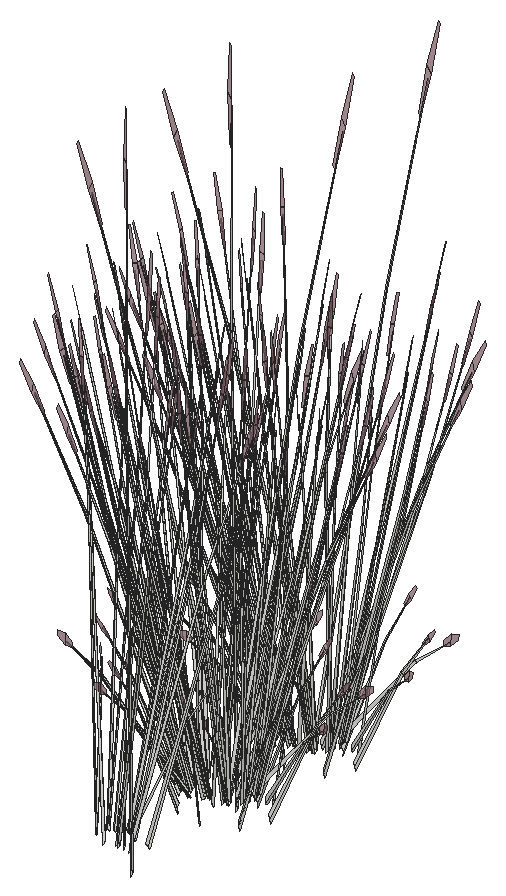
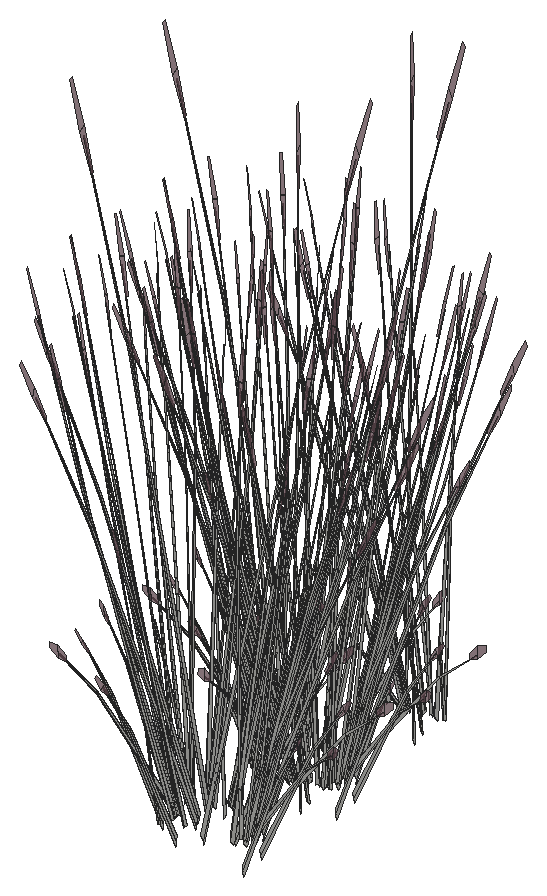
# SketchUp Ruby script. Lengths in inches.
U = 1.inch
M = Sketchup.active_model
def pt(a) = Geom::Point3d.new(a.map { |v| v * U })
def face(e, loops, mat)
  f = e.add_face(loops[0].map { |a| pt(a) })
  loops[1..].each { |l| e.add_face(l.map { |a| pt(a) }).erase! }
  f.material = f.back_material = mat if mat
  f
end
# faces: each face lists its corners as indices into pts; further lists are holes
def faces(e, pts, list, mat = nil) = list.each { |f| face(e, (f[0].is_a?(Array) ? f : [f]).map { |l| l.map { |i| pts[i] } }, mat) }
# xy, xz, yz: faces in a plane at the given z, y or x. An outline is a flat list of corners, or four numbers for a rectangle; further outlines are holes
def ring(l) = l.size == 4 ? [[l[0], l[1]], [l[2], l[1]], [l[2], l[3]], [l[0], l[3]]] : l.each_slice(2).to_a
def flat(e, list, mat, &to3) = list.each { |f| face(e, (f[0].is_a?(Array) ? f : [f]).map { |l| ring(l).map { |u, v| to3.(u, v) } }, mat) }
def xy(e, z, list, mat = nil) = flat(e, list, mat) { |x, y| [x, y, z] }
def xz(e, y, list, mat = nil) = flat(e, list, mat) { |x, z| [x, y, z] }
def yz(e, x, list, mat = nil) = flat(e, list, mat) { |y, z| [x, y, z] }
def lines(e, pts, list) = list.each { |a, b| e.add_line(pt(pts[a]), pt(pts[b])) }
# prism: a flat outline (further loops are holes) pulled along v
def prism(e, loops, v, mat = nil)
  f = face(e, loops, mat); d = Geom::Vector3d.new(v.map { |x| x * U })
  f.pushpull(f.normal.samedirection?(d) ? d.length : -d.length)
end
def box(e, o, s, mat = nil) = prism(e, [[o, [o[0] + s[0], o[1], o[2]], [o[0] + s[0], o[1] + s[1], o[2]], [o[0], o[1] + s[1], o[2]]]], [0, 0, s[2]], mat)
def at(x, y, z, deg = 0) = Geom::Transformation.translation(pt([x, y, z])) * Geom::Transformation.rotation(ORIGIN, Z_AXIS, deg.degrees)
def axes(o, x, y, z) = Geom::Transformation.new([*x, 0, *y, 0, *z, 0, *pt(o).to_a, 1])
def part(name) = M.definitions.add(name)
# library, detail: a bought-in or finely detailed component or shape, given as its bounding box
def library(name, o, s) = part(name).tap { |d| box(d.entities, o, s) }
def detail(e, o, s) = box(e.add_group.entities, o, s)
def put(e, d, t, mat = nil) = e.add_instance(d, t).tap { |i| i.material = mat if mat }
def group(e, t, mat = nil) = e.add_group.tap { |g| g.transformation = t; g.material = mat if mat }.entities
root = M.entities
M.materials.add("LightPink_Translucent").color = [144, 107, 117]
M.materials["LightPink_Translucent"].alpha = 0.75
c1 = part("blade")
p = [[2.15,0.21,22],[0,0.17,0],[0.09,0.45,0],[2.18,0.31,22],[2.29,0.31,22],[0.38,0.45,0],
  [2.48,0.24,33],[2.49,0.24,33],[2.48,0.22,33]]
faces(c1.entities,p,[[0,1,2,3],[4,5,2,3],[6,3,4,7],[8,0,3,6]])
c2 = part("seeds")
p = [[0.3,-0.1,1.38],[-0.01,-0.03,1.59],[-0.01,-0.03,0.03],[0.14,-0.07,-0.07],[0.29,-0.03,3],[0.15,0.01,3.11]]
faces(c2.entities,p,[[0,1,2,3],[1,0,4,5]],"LightPink_Translucent")
c3 = part("blade with seeds")
put(c3.entities,c1,at(0,0,0))
put(c3.entities,c2,axes([2.4,0.25,30.99],[1.5799,-0.05474,1.17369],[-0.12525,1.92788,0.29478],[-0.07173,-0.02425,1.56792]))
put(root,c3,axes([331.86,461.53,52.14],[0.12971,0.3568,-0.45151],[-0.49122,0.06241,-0.34973],[-0.14077,0.09583,0.86392]))
put(root,c3,axes([334.74,460.8,50.51],[-0.01379,-0.36791,1.24828],[0.62424,0.09537,0.52853],[-0.14764,0.20132,1.17828]))
put(root,c3,axes([334.79,462.22,52.14],[0.49824,-0.09289,-0.45151],[0.08716,0.35177,-0.34973],[0.13382,0.10081,0.86392]))
put(root,c3,axes([332.16,461.47,51.43],[0.09401,-0.13431,1.51428],[0.3944,0.27795,0.12244],[-0.17792,0.17323,0.64734]))
put(root,c3,axes([332.27,462.23,52],[-0.34164,0.20573,-0.31292],[-0.3234,-0.23491,0.40398],[-0.04921,0.11936,0.77298]))
put(root,c3,axes([331.09,462.17,52.17],[-0.01255,0.07733,1.54581],[0.35618,0.269,-0.24447],[-0.09325,0.12721,0.12397]))
put(root,c3,axes([333.25,462.4,52.45],[0.49409,-0.18193,-0.10745],[0.24281,0.32289,-0.59638],[0.06519,0.13607,0.90619]))
put(root,c3,axes([332.48,463.03,50.44],[-0.01307,-0.23234,1.01491],[0.32652,0.16572,0.74569],[-0.06422,0.11074,0.22354]))
put(root,c3,axes([332.61,462.13,52.42],[0.36145,0.26255,-0.50118],[-0.38183,0.22994,-0.3882],[-0.055,0.1334,0.95895]))
put(root,c3,axes([333.68,462.38,52.14],[0.49634,0.09796,-0.45151],[-0.17013,0.33585,-0.34973],[0.04551,0.13522,0.86392]))
put(root,c3,axes([333.96,461.69,51.43],[-0.11542,-0.12546,1.51428],[0.53333,-0.10562,0.12244],[0.12054,0.19696,0.64734]))
put(root,c3,axes([333.45,462.59,52],[-0.15222,0.30049,-0.31292],[-0.44409,-0.08764,0.40398],[0.04072,0.12098,0.77298]))
put(root,c3,axes([332.49,462.01,52.72],[-0.01314,0.36145,-0.69681],[-0.55324,-0.02428,0.08409],[-0.05838,0.15313,0.9857]))
put(root,c3,axes([332.69,468.79,51.43],[0.11542,0.12546,1.51428],[-0.53333,0.10562,0.12244],[-0.12054,-0.19696,0.64734]))
put(root,c3,axes([333.02,461.75,51.43],[-0.01236,-0.14998,1.51428],[0.53562,0.09949,0.12244],[-0.03313,0.21373,0.64734]))
put(root,c3,axes([333.57,467.96,52.17],[-0.07723,-0.05479,1.54581],[-0.51538,0.03473,-0.24447],[-0.08225,-0.13104,0.12397]))
put(root,c3,axes([333.5,462.32,52.4],[0.24099,0.31773,-0.62776],[-0.49607,0.17707,0.07576],[0.05635,0.15352,0.88802]))
put(root,c3,axes([334.11,468.88,52.4],[-0.24099,-0.31773,-0.62776],[0.49607,-0.17707,0.07576],[-0.05635,-0.15352,0.88802]))
put(root,c3,axes([333.14,463.12,52.17],[0.064,0.06292,1.54581],[0.51651,0.02472,-0.24447],[0.05194,0.13877,0.12397]))
put(root,c3,axes([335.12,469.19,52.4],[0.01314,-0.36145,-0.62776],[0.55324,0.02428,0.07576],[0.05838,-0.15313,0.88802]))
put(root,c3,axes([335.89,468.63,52.17],[-0.00487,-0.07777,1.54581],[-0.41166,-0.22476,-0.24447],[0.06364,-0.13625,0.12397]))
put(root,c3,axes([334.16,468.61,52],[0.15222,-0.30049,-0.31292],[0.44409,0.08764,0.40398],[-0.04072,-0.12098,0.77298]))
put(root,c3,axes([334.5,469.01,51.43],[-0.09401,0.13431,1.51428],[-0.3944,-0.27795,0.12244],[0.17792,-0.17323,0.64734]))
put(root,c3,axes([332.31,462.52,50.97],[0.01109,-0.20172,1.3638],[0.49896,0.10655,0.18846],[-0.04323,0.21498,0.64398]))
put(root,c3,axes([333.93,468.82,52.14],[-0.49634,-0.09796,-0.45151],[0.17013,-0.33585,-0.34973],[-0.04551,-0.13522,0.86392]))
put(root,c3,axes([334.24,467.98,50.44],[0.06477,0.22786,1.01491],[-0.35932,-0.1262,0.74569],[0.03867,-0.11667,0.22354]))
put(root,c3,axes([335.01,469.07,52.14],[-0.36145,-0.26255,-0.45151],[0.38183,-0.22994,-0.34973],[0.055,-0.1334,0.86392]))
put(root,c3,axes([334.36,468.8,52.45],[-0.49409,0.18193,-0.10745],[-0.24281,-0.32289,-0.59638],[-0.06519,-0.13607,0.90619]))
put(root,c3,axes([335.38,469.21,52.45],[-0.55492,-0.01936,-0.10745],[0.01517,-0.36657,-0.59638],[0.03855,-0.14118,0.90619]))
put(root,c3,axes([335.35,468.98,52],[0.34164,-0.20573,-0.31292],[0.3234,0.23491,0.40398],[0.04921,-0.11936,0.77298]))
put(root,c3,axes([332.39,468.25,50.44],[0.26338,0.136,1.01491],[-0.38358,0.08175,0.74569],[-0.08207,-0.10452,0.22354]))
put(root,c3,axes([333.03,468.97,52.4],[-0.43054,-0.18887,-0.62776],[0.30598,-0.33097,0.07576],[-0.15599,-0.11277,0.88802]))
put(root,c3,axes([332.88,468.72,52],[-0.07798,-0.31474,-0.31292],[0.44579,-0.08311,0.40398],[-0.11974,-0.09019,0.77298]))
put(root,c3,axes([331.92,469.18,51.43],[0.18755,0.06732,1.51428],[-0.38813,0.28243,0.12244],[-0.24191,-0.12741,0.64734]))
put(root,c3,axes([332.83,468.98,52.14],[-0.49824,0.09289,-0.45151],[-0.08716,-0.35177,-0.34973],[-0.13382,-0.10081,0.86392]))
put(root,c3,axes([335.77,469.82,52.4],[0.26374,-0.30832,-0.62776],[0.46217,0.21911,0.07576],[0.15748,-0.11171,0.88802]))
put(root,c3,axes([335.76,469.68,52.14],[-0.12971,-0.3568,-0.45151],[0.49122,-0.06241,-0.34973],[0.14077,-0.09583,0.86392]))
put(root,c3,axes([331.88,468.5625,52.17],[-0.10864,-0.00276,1.54581],[-0.34587,0.27582,-0.24447],[-0.18454,-0.05636,0.12397]))
put(root,c3,axes([335.99,469.93,52.45],[-0.46706,-0.21546,-0.10745],[0.26908,-0.31203,-0.59638],[0.13196,-0.10846,0.90619]))
put(root,c3,axes([334.06,471.11,50.9375],[0.43633,0.15757,1.33654],[-0.42745,0.33945,0.52853],[-0.19146,-0.20119,1.12046]))
put(root,c3,axes([336.36,468.97,50.44],[-0.16818,0.19891,1.01491],[-0.14456,-0.26725,0.74569],[0.1389,-0.06697,0.22354]))
put(root,c3,axes([336.12,469.72,52],[0.43951,-0.05584,-0.31292],[0.11606,0.31924,0.40398],[0.12595,-0.08575,0.77298]))
put(root,c3,axes([331.85,469.28,52],[-0.28729,-0.24465,-0.31292],[0.32804,-0.23159,0.40398],[-0.16667,-0.03524,0.77298]))
put(root,c3,axes([332.15,469.44,52.4],[-0.50473,-0.00941,-0.62776],[0.0339,-0.39618,0.07576],[-0.21383,-0.04181,0.88802]))
put(root,c3,axes([337.39,470.22,52.17],[0.07006,-0.05952,1.54581],[-0.08968,-0.3651,-0.24447],[0.1758,-0.06922,0.12397]))
put(root,c3,axes([331.98,469.52,52.14],[-0.36663,0.25884,-0.45151],[-0.32109,-0.27343,-0.34973],[-0.18628,-0.03938,0.86392]))
put(root,c3,axes([331.16,469.86,50.44],[0.32236,-0.02796,1.01491],[-0.20448,0.24636,0.74569],[-0.1593,-0.03696,0.22354]))
put(root,c3,axes([332.18,469.25,52.45],[-0.02704,0.39739,-0.10745],[-0.51189,-0.01086,-0.59638],[-0.19715,-0.0276,0.90619]))
put(root,c3,axes([336.01,470.78,52.45],[-0.25405,-0.35383,-0.10745],[0.45089,-0.17388,-0.59638],[0.19001,-0.04668,0.90619]))
put(root,c3,axes([335.98,470.47,52.14],[0.13679,-0.35544,-0.45151],[0.46898,0.12183,-0.34973],[0.18882,-0.03259,0.86392]))
put(root,c3,axes([331.52,469.8,51.43],[0.20943,-0.00885,1.51428],[-0.13893,0.38357,0.12244],[-0.29846,-0.02372,0.64734]))
put(root,c3,axes([335.9,470.6,52.4],[0.44368,-0.17257,-0.62776],[0.24726,0.35524,0.07576],[0.21437,-0.04035,0.88802]))
put(root,c3,axes([336.27,470.63,52],[0.41962,0.10901,-0.31292],[-0.12239,0.31802,0.40398],[0.16894,-0.02916,0.77298]))
put(root,c3,axes([331.34,470.125,52],[-0.41962,-0.10901,-0.31292],[0.12239,-0.31802,0.40398],[-0.16894,0.02916,0.77298]))
put(root,c3,axes([335.13,470.24,51.43],[-0.20943,0.00885,1.51428],[0.13893,-0.38357,0.12244],[0.29846,0.02372,0.64734]))
put(root,c3,axes([332.62,470.07,50.95],[0.14352,-0.05653,1.56454],[0.04949,0.39467,0.12244],[-0.31087,0.05237,0.55918]))
put(root,c3,axes([337.16,470.7,50.44],[-0.31197,0.06451,1.01491],[0.14684,-0.26661,0.74569],[0.1655,0.01824,0.22354]))
put(root,c3,axes([331.08,470.34,52.17],[-0.08245,0.05073,1.54581],[0.00701,0.37067,-0.24447],[-0.18899,0.0482,0.12397]))
put(root,c3,axes([331.63,470.29,52.14],[-0.13679,0.35544,-0.45151],[-0.46898,-0.12183,-0.34973],[-0.18882,0.03259,0.86392]))
put(root,c3,axes([331.61,469.99,52.45],[0.25405,0.35383,-0.10745],[-0.45089,0.17388,-0.59638],[-0.19001,0.04668,0.90619]))
put(root,c3,axes([336.62,471.52,51.47],[-0.09664,-0.32847,-0.03085],[0.45676,-0.07551,-0.13989],[0.09538,0.02082,0.4614]))
put(root,c3,axes([335.4375,471.51,52.45],[0.02704,-0.39739,-0.10745],[0.51189,0.01086,-0.59638],[0.19715,0.0276,0.90619]))
put(root,c3,axes([335.88,471.27,52.17],[0.10831,-0.00661,1.54581],[0.29709,-0.30358,-0.24447],[0.19266,0.04007,0.12397]))
put(root,c3,axes([331.61,470.47,51.43],[0.17519,-0.08265,1.51428],[0.14749,0.38193,0.12244],[-0.27504,0.08632,0.64734]))
put(root,c3,axes([335.46,471.32,52.4],[0.50473,0.00941,-0.62776],[-0.0339,0.39618,0.07576],[0.21383,0.04181,0.88802]))
put(root,c3,axes([330.7,471.81,50.44],[0.21042,-0.1771,1.01491],[0.08303,0.28036,0.74569],[-0.15207,0.0502,0.22354]))
put(root,c3,axes([335.77,471.48,52],[0.28729,0.24465,-0.31292],[-0.32804,0.23159,0.40398],[0.16667,0.03524,0.77298]))
put(root,c3,axes([331.49,471.04,52],[-0.43951,0.05584,-0.31292],[-0.11606,-0.31924,0.40398],[-0.12595,0.08575,0.77298]))
put(root,c3,axes([334.73,470.86,51.43],[-0.18755,-0.06732,1.51428],[0.38813,-0.28243,0.12244],[0.24191,0.12741,0.64734]))
put(root,c3,axes([334.77,469.97,51.95],[-0.4363,-0.20303,1.22187],[0.46069,-0.31611,0.5272],[0.14077,0.1905,1.18105]))
put(root,c3,axes([331.625,470.83,52.45],[0.46706,0.21546,-0.10745],[-0.26908,0.31203,-0.59638],[-0.13196,0.10846,0.90619]))
put(root,c3,axes([335.43,471.62,50.44],[-0.28429,-0.11236,1.01491],[0.36709,-0.11416,0.74569],[0.09901,0.0967,0.22354]))
put(root,c3,axes([334.43,471.94,52.45],[0.30087,-0.33447,-0.10745],[0.43572,0.19269,-0.59638],[0.15146,0.0945,0.90619]))
put(root,c3,axes([332.69,476.59,51.43],[0.11542,0.12546,1.51428],[-0.53333,0.10562,0.12244],[-0.12054,-0.19696,0.64734]))
put(root,c3,axes([332.25,470.73,51.43],[0.12611,-0.12006,1.51428],[0.31843,0.32408,0.12244],[-0.2184,0.14759,0.64734]))
put(root,c3,axes([333.57,475.76,52.17],[-0.07723,-0.05479,1.54581],[-0.51538,0.03473,-0.24447],[-0.08225,-0.13104,0.12397]))
put(root,c3,axes([331.86,471.08,52.14],[0.12971,0.3568,-0.45151],[-0.49122,0.06241,-0.34973],[-0.14077,0.09583,0.86392]))
put(root,c3,axes([334.11,476.68,52.4],[-0.24099,-0.31773,-0.62776],[0.49607,-0.17707,0.07576],[-0.05635,-0.15352,0.88802]))
put(root,c3,axes([334.74,470.36,50.51],[-0.01379,-0.36791,1.24828],[0.62424,0.09537,0.52853],[-0.14764,0.20132,1.17828]))
put(root,c3,axes([334.79,471.78,52.14],[0.49824,-0.09289,-0.45151],[0.08716,0.35177,-0.34973],[0.13382,0.10081,0.86392]))
put(root,c3,axes([335.12,476.99,52.4],[0.01314,-0.36145,-0.62776],[0.55324,0.02428,0.07576],[0.05838,-0.15313,0.88802]))
put(root,c3,axes([335.89,476.43,52.17],[-0.00487,-0.07777,1.54581],[-0.41166,-0.22476,-0.24447],[0.06364,-0.13625,0.12397]))
put(root,c3,axes([334.16,476.41,52],[0.15222,-0.30049,-0.31292],[0.44409,0.08764,0.40398],[-0.04072,-0.12098,0.77298]))
put(root,c3,axes([334.5,476.81,51.43],[-0.09401,0.13431,1.51428],[-0.3944,-0.27795,0.12244],[0.17792,-0.17323,0.64734]))
put(root,c3,axes([333.93,476.62,52.14],[-0.49634,-0.09796,-0.45151],[0.17013,-0.33585,-0.34973],[-0.04551,-0.13522,0.86392]))
put(root,c3,axes([334.24,475.78,50.44],[0.06477,0.22786,1.01491],[-0.35932,-0.1262,0.74569],[0.03867,-0.11667,0.22354]))
put(root,c3,axes([332.16,471.03,51.43],[0.09401,-0.13431,1.51428],[0.3944,0.27795,0.12244],[-0.17792,0.17323,0.64734]))
put(root,c3,axes([335.01,476.87,52.14],[-0.36145,-0.26255,-0.45151],[0.38183,-0.22994,-0.34973],[0.055,-0.1334,0.86392]))
put(root,c3,axes([332.27,471.78,52],[-0.34164,0.20573,-0.31292],[-0.3234,-0.23491,0.40398],[-0.04921,0.11936,0.77298]))
put(root,c3,axes([331.09,471.72,52.17],[-0.01255,0.07733,1.54581],[0.35618,0.269,-0.24447],[-0.09325,0.12721,0.12397]))
put(root,c3,axes([333.25,471.96,52.45],[0.49409,-0.18193,-0.10745],[0.24281,0.32289,-0.59638],[0.06519,0.13607,0.90619]))
put(root,c3,axes([332.48,472.58,50.44],[-0.01307,-0.23234,1.01491],[0.32652,0.16572,0.74569],[-0.06422,0.11074,0.22354]))
put(root,c3,axes([334.36,476.6,52.45],[-0.49409,0.18193,-0.10745],[-0.24281,-0.32289,-0.59638],[-0.06519,-0.13607,0.90619]))
put(root,c3,axes([335.38,477.01,52.45],[-0.55492,-0.01936,-0.10745],[0.01517,-0.36657,-0.59638],[0.03855,-0.14118,0.90619]))
put(root,c3,axes([335.35,476.77,52],[0.34164,-0.20573,-0.31292],[0.3234,0.23491,0.40398],[0.04921,-0.11936,0.77298]))
put(root,c3,axes([332.39,476.05,50.44],[0.26338,0.136,1.01491],[-0.38358,0.08175,0.74569],[-0.08207,-0.10452,0.22354]))
put(root,c3,axes([333.03,476.77,52.4],[-0.43054,-0.18887,-0.62776],[0.30598,-0.33097,0.07576],[-0.15599,-0.11277,0.88802]))
put(root,c3,axes([332.88,476.52,52],[-0.07798,-0.31474,-0.31292],[0.44579,-0.08311,0.40398],[-0.11974,-0.09019,0.77298]))
put(root,c3,axes([332.61,471.6875,52.42],[0.36145,0.26255,-0.50118],[-0.38183,0.22994,-0.3882],[-0.055,0.1334,0.95895]))
put(root,c3,axes([333.68,471.94,52.14],[0.49634,0.09796,-0.45151],[-0.17013,0.33585,-0.34973],[0.04551,0.13522,0.86392]))
put(root,c3,axes([333.96,471.25,51.43],[-0.11542,-0.12546,1.51428],[0.53333,-0.10562,0.12244],[0.12054,0.19696,0.64734]))
put(root,c3,axes([333.45,472.15,52],[-0.15222,0.30049,-0.31292],[-0.44409,-0.08764,0.40398],[0.04072,0.12098,0.77298]))
put(root,c3,axes([331.92,476.98,51.43],[0.18755,0.06732,1.51428],[-0.38813,0.28243,0.12244],[-0.24191,-0.12741,0.64734]))
put(root,c3,axes([332.49,471.57,52.72],[-0.01314,0.36145,-0.69681],[-0.55324,-0.02428,0.08409],[-0.05838,0.15313,0.9857]))
put(root,c3,axes([333.02,471.31,51.43],[-0.01236,-0.14998,1.51428],[0.53562,0.09949,0.12244],[-0.03313,0.21373,0.64734]))
put(root,c3,axes([332.83,476.78,52.14],[-0.49824,0.09289,-0.45151],[-0.08716,-0.35177,-0.34973],[-0.13382,-0.10081,0.86392]))
put(root,c3,axes([333.5,471.875,52.4],[0.24099,0.31773,-0.62776],[-0.49607,0.17707,0.07576],[0.05635,0.15352,0.88802]))
put(root,c3,axes([335.77,477.62,52.4],[0.26374,-0.30832,-0.62776],[0.46217,0.21911,0.07576],[0.15748,-0.11171,0.88802]))
put(root,c3,axes([335.76,477.48,52.14],[-0.12971,-0.3568,-0.45151],[0.49122,-0.06241,-0.34973],[0.14077,-0.09583,0.86392]))
put(root,c3,axes([333.14,472.68,52.17],[0.064,0.06292,1.54581],[0.51651,0.02472,-0.24447],[0.05194,0.13877,0.12397]))
put(root,c3,axes([331.88,476.36,52.17],[-0.10864,-0.00276,1.54581],[-0.34587,0.27582,-0.24447],[-0.18454,-0.05636,0.12397]))
put(root,c3,axes([335.99,477.73,52.45],[-0.46706,-0.21546,-0.10745],[0.26908,-0.31203,-0.59638],[0.13196,-0.10846,0.90619]))
put(root,c3,axes([334.06,478.91,50.9375],[0.43633,0.15757,1.33654],[-0.42745,0.33945,0.52853],[-0.19146,-0.20119,1.12046]))
put(root,c3,axes([332.31,472.07,50.97],[0.01109,-0.20172,1.3638],[0.49896,0.10655,0.18846],[-0.04323,0.21498,0.64398]))
put(root,c3,axes([336.36,476.77,50.44],[-0.16818,0.19891,1.01491],[-0.14456,-0.26725,0.74569],[0.1389,-0.06697,0.22354]))
put(root,c3,axes([336.12,477.51,52],[0.43951,-0.05584,-0.31292],[0.11606,0.31924,0.40398],[0.12595,-0.08575,0.77298]))
put(root,c3,axes([331.85,477.07,52],[-0.28729,-0.24465,-0.31292],[0.32804,-0.23159,0.40398],[-0.16667,-0.03524,0.77298]))
put(root,c3,axes([332.15,477.24,52.4],[-0.50473,-0.00941,-0.62776],[0.0339,-0.39618,0.07576],[-0.21383,-0.04181,0.88802]))
put(root,c3,axes([337.39,478.02,52.17],[0.07006,-0.05952,1.54581],[-0.08968,-0.3651,-0.24447],[0.1758,-0.06922,0.12397]))
put(root,c3,axes([331.98,477.32,52.14],[-0.36663,0.25884,-0.45151],[-0.32109,-0.27343,-0.34973],[-0.18628,-0.03938,0.86392]))
put(root,c3,axes([331.16,477.66,50.44],[0.32236,-0.02796,1.01491],[-0.20448,0.24636,0.74569],[-0.1593,-0.03696,0.22354]))
put(root,c3,axes([332.18,477.05,52.45],[-0.02704,0.39739,-0.10745],[-0.51189,-0.01086,-0.59638],[-0.19715,-0.0276,0.90619]))
put(root,c3,axes([336.01,478.57,52.45],[-0.25405,-0.35383,-0.10745],[0.45089,-0.17388,-0.59638],[0.19001,-0.04668,0.90619]))
put(root,c3,axes([335.98,478.27,52.14],[0.13679,-0.35544,-0.45151],[0.46898,0.12183,-0.34973],[0.18882,-0.03259,0.86392]))
put(root,c3,axes([331.52,477.59,51.43],[0.20943,-0.00885,1.51428],[-0.13893,0.38357,0.12244],[-0.29846,-0.02372,0.64734]))
put(root,c3,axes([335.9,478.4,52.4],[0.44368,-0.17257,-0.62776],[0.24726,0.35524,0.07576],[0.21437,-0.04035,0.88802]))
put(root,c3,axes([336.27,478.43,52],[0.41962,0.10901,-0.31292],[-0.12239,0.31802,0.40398],[0.16894,-0.02916,0.77298]))
put(root,c3,axes([331.34,477.92,52],[-0.41962,-0.10901,-0.31292],[0.12239,-0.31802,0.40398],[-0.16894,0.02916,0.77298]))
put(root,c3,axes([335.13,478.04,51.43],[-0.20943,0.00885,1.51428],[0.13893,-0.38357,0.12244],[0.29846,0.02372,0.64734]))
put(root,c3,axes([332.62,477.87,50.95],[0.14352,-0.05653,1.56454],[0.04949,0.39467,0.12244],[-0.31087,0.05237,0.55918]))
put(root,c3,axes([337.16,478.5,50.44],[-0.31197,0.06451,1.01491],[0.14684,-0.26661,0.74569],[0.1655,0.01824,0.22354]))
put(root,c3,axes([331.08,478.14,52.17],[-0.08245,0.05073,1.54581],[0.00701,0.37067,-0.24447],[-0.18899,0.0482,0.12397]))
put(root,c3,axes([331.63,478.09,52.14],[-0.13679,0.35544,-0.45151],[-0.46898,-0.12183,-0.34973],[-0.18882,0.03259,0.86392]))
put(root,c3,axes([331.61,477.78,52.45],[0.25405,0.35383,-0.10745],[-0.45089,0.17388,-0.59638],[-0.19001,0.04668,0.90619]))
put(root,c3,axes([336.62,479.32,51.47],[-0.09664,-0.32847,-0.03085],[0.45676,-0.07551,-0.13989],[0.09538,0.02082,0.4614]))
put(root,c3,axes([335.4375,479.31,52.45],[0.02704,-0.39739,-0.10745],[0.51189,0.01086,-0.59638],[0.19715,0.0276,0.90619]))
put(root,c3,axes([335.88,479.07,52.17],[0.10831,-0.00661,1.54581],[0.29709,-0.30358,-0.24447],[0.19266,0.04007,0.12397]))
put(root,c3,axes([331.61,478.27,51.43],[0.17519,-0.08265,1.51428],[0.14749,0.38193,0.12244],[-0.27504,0.08632,0.64734]))
put(root,c3,axes([335.46,479.12,52.4],[0.50473,0.00941,-0.62776],[-0.0339,0.39618,0.07576],[0.21383,0.04181,0.88802]))
put(root,c3,axes([330.7,479.61,50.44],[0.21042,-0.1771,1.01491],[0.08303,0.28036,0.74569],[-0.15207,0.0502,0.22354]))
put(root,c3,axes([335.77,479.28,52],[0.28729,0.24465,-0.31292],[-0.32804,0.23159,0.40398],[0.16667,0.03524,0.77298]))
put(root,c3,axes([331.49,478.84,52],[-0.43951,0.05584,-0.31292],[-0.11606,-0.31924,0.40398],[-0.12595,0.08575,0.77298]))
put(root,c3,axes([334.73,478.65,51.43],[-0.18755,-0.06732,1.51428],[0.38813,-0.28243,0.12244],[0.24191,0.12741,0.64734]))
put(root,c3,axes([334.77,477.77,51.95],[-0.4363,-0.20303,1.22187],[0.46069,-0.31611,0.5272],[0.14077,0.1905,1.18105]))
put(root,c3,axes([331.625,478.62,52.45],[0.46706,0.21546,-0.10745],[-0.26908,0.31203,-0.59638],[-0.13196,0.10846,0.90619]))
put(root,c3,axes([335.43,479.42,50.44],[-0.28429,-0.11236,1.01491],[0.36709,-0.11416,0.74569],[0.09901,0.0967,0.22354]))
put(root,c3,axes([334.43,479.74,52.45],[0.30087,-0.33447,-0.10745],[0.43572,0.19269,-0.59638],[0.15146,0.0945,0.90619]))
put(root,c3,axes([332.25,478.53,51.43],[0.12611,-0.12006,1.51428],[0.31843,0.32408,0.12244],[-0.2184,0.14759,0.64734]))
